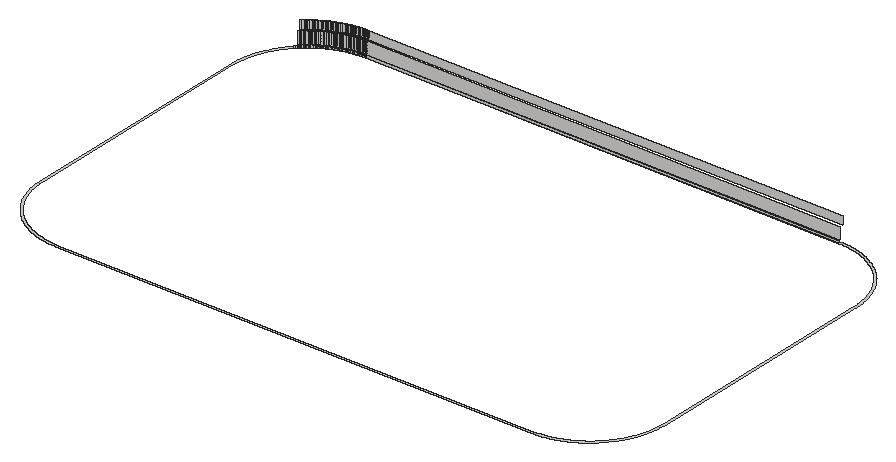
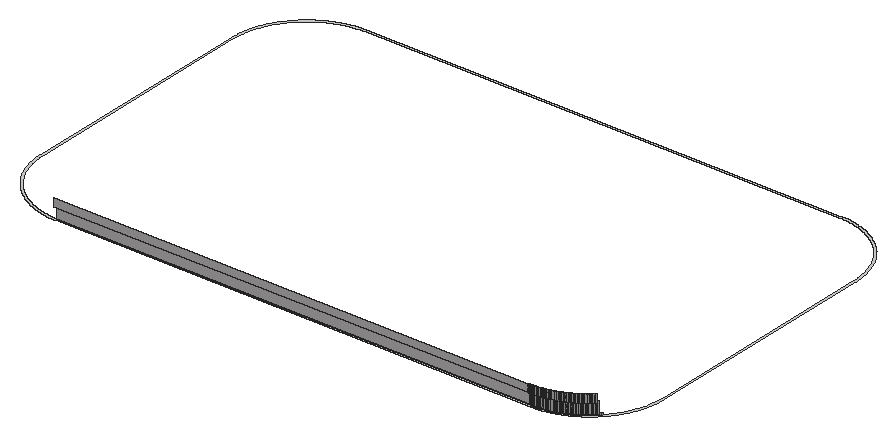
# SketchUp Ruby script. Lengths in inches.
U = 1.inch
M = Sketchup.active_model
def pt(a) = Geom::Point3d.new(a.map { |v| v * U })
def face(e, loops, mat)
  f = e.add_face(loops[0].map { |a| pt(a) })
  loops[1..].each { |l| e.add_face(l.map { |a| pt(a) }).erase! }
  f.material = f.back_material = mat if mat
  f
end
# faces: each face lists its corners as indices into pts; further lists are holes
def faces(e, pts, list, mat = nil) = list.each { |f| face(e, (f[0].is_a?(Array) ? f : [f]).map { |l| l.map { |i| pts[i] } }, mat) }
# xy, xz, yz: faces in a plane at the given z, y or x. An outline is a flat list of corners, or four numbers for a rectangle; further outlines are holes
def ring(l) = l.size == 4 ? [[l[0], l[1]], [l[2], l[1]], [l[2], l[3]], [l[0], l[3]]] : l.each_slice(2).to_a
def flat(e, list, mat, &to3) = list.each { |f| face(e, (f[0].is_a?(Array) ? f : [f]).map { |l| ring(l).map { |u, v| to3.(u, v) } }, mat) }
def xy(e, z, list, mat = nil) = flat(e, list, mat) { |x, y| [x, y, z] }
def xz(e, y, list, mat = nil) = flat(e, list, mat) { |x, z| [x, y, z] }
def yz(e, x, list, mat = nil) = flat(e, list, mat) { |y, z| [x, y, z] }
def lines(e, pts, list) = list.each { |a, b| e.add_line(pt(pts[a]), pt(pts[b])) }
# prism: a flat outline (further loops are holes) pulled along v
def prism(e, loops, v, mat = nil)
  f = face(e, loops, mat); d = Geom::Vector3d.new(v.map { |x| x * U })
  f.pushpull(f.normal.samedirection?(d) ? d.length : -d.length)
end
def box(e, o, s, mat = nil) = prism(e, [[o, [o[0] + s[0], o[1], o[2]], [o[0] + s[0], o[1] + s[1], o[2]], [o[0], o[1] + s[1], o[2]]]], [0, 0, s[2]], mat)
def at(x, y, z, deg = 0) = Geom::Transformation.translation(pt([x, y, z])) * Geom::Transformation.rotation(ORIGIN, Z_AXIS, deg.degrees)
def axes(o, x, y, z) = Geom::Transformation.new([*x, 0, *y, 0, *z, 0, *pt(o).to_a, 1])
def part(name) = M.definitions.add(name)
# library, detail: a bought-in or finely detailed component or shape, given as its bounding box
def library(name, o, s) = part(name).tap { |d| box(d.entities, o, s) }
def detail(e, o, s) = box(e.add_group.entities, o, s)
def put(e, d, t, mat = nil) = e.add_instance(d, t).tap { |i| i.material = mat if mat }
def group(e, t, mat = nil) = e.add_group.tap { |g| g.transformation = t; g.material = mat if mat }.entities
root = M.entities
M.materials.add("[Quartz Light Brown]").color = [215, 212, 212]
xy(root,486,[[[224.5,282.7,464.5,282.7,464.99,282.71,465.99,282.75,466.49,282.78,466.98,282.82,467.48,282.86,467.97,282.91,468.47,282.96,468.96,283.03,469.45,283.09,469.94,283.17,470.44,283.25,470.92,283.34,471.41,283.43,471.9,283.53,472.39,283.64,472.87,283.75,473.35,283.87,473.84,284,474.31,284.13,475.27,284.41,475.74,284.5625,476.21,284.72,476.68,284.88,477.62,285.22,478.08,285.41,478.54,285.59,479.46,285.99,479.91,286.19,480.36,286.4,480.81,286.62,481.25,286.84,481.69,287.07,482.57,287.55,483,287.79,483.43,288.04,483.85,288.3,484.28,288.5625,484.7,288.83,485.11,289.11,485.52,289.38,486.34,289.96,486.74,290.25,487.13,290.55,487.53,290.86,487.91,291.17,488.3,291.49,489.06,292.13,489.43,292.46,489.79,292.8,490.16,293.14,490.52,293.48,491.22,294.18,491.5625,294.54,491.9,294.91,492.24,295.27,492.57,295.65,492.9,296.02,493.22,296.4,494.15,297.57,494.45,297.96,494.74,298.37,495.03,298.77,495.32,299.18,495.6,299.59,495.87,300,496.14,300.42,496.4,300.85,496.66,301.27,496.91,301.7,497.15,302.13,497.4,302.57,497.86,303.45,498.08,303.89,498.3,304.34,498.51,304.79,498.71,305.25,498.91,305.7,499.11,306.16,499.29,306.62,499.48,307.08,499.82,308.02,500.14,308.96,500.29,309.43,500.44,309.91,500.57,310.39,500.71,310.87,500.95,311.83,501.0625,312.31,501.17,312.8,501.27,313.29,501.45,314.27,501.61,315.25,501.67,315.74,501.74,316.23,501.79,316.73,501.84,317.22,501.92,318.22,501.95,318.71,501.99,319.71,502,320.2,502,441.2,501.99,441.7,501.97,442.19,501.95,442.69,501.92,443.1875,501.88,443.68,501.84,444.18,501.79,444.67,501.74,445.17,501.67,445.66,501.61,446.15,501.53,446.65,501.45,447.14,501.27,448.11,501.17,448.6,501.0625,449.09,500.95,449.57,500.83,450.05,500.71,450.54,500.57,451.02,500.44,451.49,500.29,451.97,500.14,452.44,499.98,452.92,499.82,453.39,499.65,453.85,499.48,454.32,499.29,454.78,499.11,455.24,498.71,456.16,498.51,456.61,498.3,457.06,498.08,457.51,497.86,457.95,497.4,458.83,497.15,459.27,496.91,459.7,496.66,460.13,496.4,460.56,496.14,460.98,495.87,461.4,495.6,461.8125,495.32,462.22,494.74,463.04,494.45,463.4375,494.15,463.83,493.84,464.23,493.53,464.62,493.22,465,492.9,465.38,492.57,465.76,492.24,466.13,491.9,466.5,491.5625,466.86,491.22,467.22,490.52,467.92,490.16,468.27,489.79,468.61,489.43,468.94,489.06,469.27,488.68,469.6,488.3,469.92,487.91,470.23,487.53,470.54,487.13,470.85,486.74,471.15,486.34,471.44,485.52,472.02,485.11,472.3,484.7,472.57,484.28,472.84,483.85,473.1,483.43,473.36,482.57,473.86,482.13,474.1,481.25,474.56,480.81,474.78,480.36,475,479.46,475.42,479,475.62,478.08,476,477.62,476.18,476.68,476.52,475.74,476.84,475.27,476.99,474.79,477.14,474.31,477.27,473.84,477.41,473.35,477.53,472.87,477.65,472.39,477.76,471.9,477.87,471.41,477.97,470.92,478.06,470.44,478.15,469.94,478.23,469.45,478.31,468.96,478.375,468.47,478.4375,467.97,478.49,467.48,478.54,466.98,478.58,466.49,478.62,465.99,478.65,465.49,478.67,464.99,478.6875,464.5,478.7,224.5,478.7,224.01,478.6875,223.51,478.67,223.01,478.65,222.51,478.62,222.02,478.58,221.52,478.54,221.03,478.49,220.53,478.4375,220.04,478.375,219.55,478.31,219.06,478.23,218.56,478.15,218.08,478.06,217.59,477.97,217.1,477.87,216.61,477.76,216.13,477.65,215.65,477.53,215.16,477.41,214.69,477.27,214.21,477.14,213.73,476.99,213.26,476.84,212.32,476.52,211.38,476.18,210.92,476,210,475.62,209.54,475.42,208.64,475,208.19,474.78,207.75,474.56,206.87,474.1,206.43,473.86,205.57,473.36,205.15,473.1,204.72,472.84,204.3,472.57,203.89,472.3,203.48,472.02,202.66,471.44,202.26,471.15,201.87,470.85,201.47,470.54,201.09,470.23,200.7,469.92,200.32,469.6,199.94,469.27,199.57,468.94,199.21,468.61,198.84,468.27,198.48,467.92,197.78,467.22,197.4375,466.86,197.1,466.5,196.76,466.13,196.43,465.76,196.1,465.38,195.78,465,195.47,464.62,195.16,464.23,194.85,463.83,194.55,463.4375,194.26,463.04,193.68,462.22,193.4,461.8125,193.13,461.4,192.86,460.98,192.6,460.56,192.34,460.13,192.09,459.7,191.85,459.27,191.6,458.83,191.14,457.95,190.92,457.51,190.7,457.06,190.49,456.61,190.29,456.16,189.89,455.24,189.71,454.78,189.52,454.32,189.35,453.85,189.18,453.39,189.02,452.92,188.86,452.44,188.71,451.97,188.56,451.49,188.43,451.02,188.29,450.54,188.17,450.05,188.05,449.57,187.9375,449.09,187.83,448.6,187.73,448.11,187.55,447.14,187.47,446.65,187.39,446.15,187.33,445.66,187.26,445.17,187.21,444.67,187.16,444.18,187.12,443.68,187.08,443.1875,187.05,442.69,187.03,442.19,187.01,441.7,187,441.2,187,320.2,187.01,319.71,187.05,318.71,187.08,318.22,187.16,317.22,187.21,316.73,187.26,316.23,187.33,315.74,187.39,315.25,187.55,314.27,187.73,313.29,187.83,312.8,187.9375,312.31,188.05,311.83,188.29,310.87,188.43,310.39,188.56,309.91,188.71,309.43,188.86,308.96,189.18,308.02,189.52,307.08,189.71,306.62,189.89,306.16,190.09,305.7,190.29,305.25,190.49,304.79,190.7,304.34,190.92,303.89,191.14,303.45,191.6,302.57,191.85,302.13,192.09,301.7,192.34,301.27,192.6,300.85,192.86,300.42,193.13,300,193.4,299.59,193.68,299.18,193.97,298.77,194.26,298.37,194.55,297.96,194.85,297.57,195.78,296.4,196.1,296.02,196.43,295.65,196.76,295.27,197.1,294.91,197.4375,294.54,197.78,294.18,198.48,293.48,198.84,293.14,199.21,292.8,199.57,292.46,199.94,292.13,200.7,291.49,201.09,291.17,201.47,290.86,201.87,290.55,202.26,290.25,202.66,289.96,203.48,289.38,203.89,289.11,204.3,288.83,204.72,288.5625,205.15,288.3,205.57,288.04,206,287.79,206.43,287.55,207.31,287.07,207.75,286.84,208.19,286.62,208.64,286.4,209.09,286.19,209.54,285.99,210.46,285.59,210.92,285.41,211.38,285.22,212.32,284.88,212.79,284.72,213.26,284.5625,213.73,284.41,214.69,284.13,215.16,284,215.65,283.87,216.13,283.75,216.61,283.64,217.1,283.53,217.59,283.43,218.08,283.34,218.56,283.25,219.06,283.17,219.55,283.09,220.04,283.03,220.53,282.96,221.03,282.91,221.52,282.86,222.02,282.82,222.51,282.78,223.01,282.75,224.01,282.71],[224.52,283.7,224.03,283.71,223.55,283.73,223.0625,283.75,222.58,283.78,222.1,283.82,221.61,283.86,221.13,283.9,219.69,284.08,218.73,284.24,218.26,284.32,217.78,284.41,217.31,284.51,216.83,284.61,216.36,284.72,215.42,284.96,214.96,285.09,214.49,285.22,214.03,285.37,213.57,285.51,213.11,285.66,212.65,285.82,212.19,285.99,211.74,286.16,210.84,286.52,210.39,286.71,209.95,286.9,209.51,287.1,209.07,287.31,208.64,287.52,208.2,287.73,207.77,287.96,207.35,288.18,206.92,288.42,206.08,288.9,205.67,289.15,204.85,289.67,204.44,289.9375,204.04,290.21,203.65,290.49,203.25,290.77,202.86,291.05,202.48,291.35,202.09,291.64,201.72,291.95,201.34,292.25,200.97,292.57,200.6,292.88,200.24,293.2,199.88,293.53,199.53,293.86,199.18,294.2,198.5,294.88,198.16,295.23,197.83,295.59,197.5,295.94,197.18,296.31,196.86,296.67,196.55,297.04,196.25,297.42,195.94,297.79,195.65,298.18,195.35,298.5625,195.07,298.95,194.78,299.35,194.51,299.74,194.24,300.14,193.97,300.55,193.45,301.37,193.2,301.78,192.72,302.62,192.48,303.05,192.26,303.47,192.03,303.9,191.82,304.34,191.6,304.77,191.2,305.65,191,306.1,190.82,306.54,190.63,306.99,190.29,307.89,190.12,308.35,189.96,308.81,189.8125,309.27,189.66,309.73,189.52,310.19,189.39,310.66,189.26,311.125,189.14,311.59,189.02,312.0625,188.91,312.54,188.71,313.48,188.53,314.44,188.46,314.91,188.38,315.39,188.2,316.83,188.16,317.32,188.11,317.8,188.05,318.76,188.03,319.25,188.01,319.73,188,320.22,188,441.19,188.01,441.67,188.03,442.15,188.05,442.64,188.11,443.6,188.16,444.09,188.2,444.57,188.38,446.01,188.46,446.49,188.53,446.97,188.62,447.44,188.71,447.92,188.81,448.39,188.91,448.87,189.02,449.34,189.26,450.28,189.39,450.74,189.52,451.21,189.66,451.67,189.8125,452.13,189.96,452.59,190.12,453.05,190.29,453.51,190.63,454.41,190.82,454.86,191,455.31,191.6,456.63,191.82,457.07,192.03,457.5,192.26,457.93,192.48,458.36,193.2,459.62,193.45,460.03,193.97,460.85,194.24,461.26,194.78,462.06,195.07,462.45,195.35,462.84,195.65,463.23,195.94,463.61,196.25,463.99,196.55,464.36,196.86,464.73,197.18,465.1,197.5,465.46,197.83,465.82,198.16,466.17,198.5,466.52,199.18,467.2,199.53,467.54,199.88,467.87,200.24,468.2,200.6,468.52,200.97,468.84,201.34,469.15,201.72,469.46,202.09,469.76,202.48,470.06,202.86,470.35,203.25,470.63,203.65,470.92,204.04,471.19,204.44,471.47,205.67,472.25,206.08,472.5,206.92,472.98,207.35,473.22,207.77,473.45,208.2,473.67,208.64,473.89,209.07,474.1,210.39,474.7,210.84,474.88,211.29,475.07,212.19,475.41,212.65,475.58,213.11,475.74,214.03,476.04,214.49,476.18,214.96,476.3125,215.42,476.44,215.89,476.5625,216.36,476.68,216.83,476.79,217.31,476.89,217.78,476.99,218.26,477.08,218.73,477.17,219.21,477.25,219.69,477.32,221.13,477.5,221.61,477.55,222.1,477.59,222.58,477.62,223.0625,477.65,223.55,477.67,224.03,477.6875,224.52,477.7,464.48,477.7,464.97,477.6875,465.45,477.67,465.9375,477.65,466.42,477.62,466.9,477.59,467.39,477.55,467.87,477.5,469.31,477.32,469.79,477.25,470.27,477.17,470.74,477.08,471.22,476.99,471.69,476.89,472.17,476.79,472.64,476.68,473.11,476.5625,473.58,476.44,474.04,476.3125,474.51,476.18,474.97,476.04,475.89,475.74,476.35,475.58,476.81,475.41,477.71,475.07,478.16,474.88,478.61,474.7,479.93,474.1,480.36,473.89,480.8,473.67,481.23,473.45,481.65,473.22,482.08,472.98,482.92,472.5,483.33,472.25,484.56,471.47,484.96,471.19,485.35,470.92,485.75,470.63,486.14,470.35,486.52,470.06,486.91,469.76,487.28,469.46,487.66,469.15,488.03,468.84,488.4,468.52,488.76,468.2,489.12,467.87,489.47,467.54,489.82,467.2,490.5,466.52,490.84,466.17,491.17,465.82,491.5,465.46,491.82,465.1,492.14,464.73,492.45,464.36,492.75,463.99,493.06,463.61,493.35,463.23,493.65,462.84,493.93,462.45,494.22,462.06,494.76,461.26,495.03,460.85,495.55,460.03,495.8,459.62,496.52,458.36,496.74,457.93,496.97,457.5,497.18,457.07,497.4,456.63,498,455.31,498.18,454.86,498.37,454.41,498.71,453.51,498.88,453.05,499.04,452.59,499.1875,452.13,499.34,451.67,499.48,451.21,499.61,450.74,499.74,450.28,499.98,449.34,500.09,448.87,500.19,448.39,500.29,447.92,500.38,447.44,500.47,446.97,500.54,446.49,500.62,446.01,500.8,444.57,500.84,444.09,500.89,443.6,500.95,442.64,500.97,442.15,500.99,441.67,501,441.19,501,320.22,500.99,319.73,500.97,319.25,500.95,318.76,500.89,317.8,500.84,317.32,500.8,316.83,500.62,315.39,500.54,314.91,500.47,314.44,500.29,313.48,500.09,312.54,499.98,312.0625,499.86,311.59,499.74,311.125,499.61,310.66,499.48,310.19,499.34,309.73,499.1875,309.27,499.04,308.81,498.88,308.35,498.71,307.89,498.37,306.99,498.18,306.54,498,306.1,497.8,305.65,497.4,304.77,497.18,304.34,496.97,303.9,496.74,303.47,496.52,303.05,496.28,302.62,495.8,301.78,495.55,301.37,495.03,300.55,494.76,300.14,494.49,299.74,494.22,299.35,493.93,298.95,493.65,298.5625,493.35,298.18,493.06,297.79,492.75,297.42,492.45,297.04,492.14,296.67,491.82,296.31,491.5,295.94,491.17,295.59,490.84,295.23,490.5,294.88,489.82,294.2,489.47,293.86,489.12,293.53,488.76,293.2,488.4,292.88,488.03,292.57,487.66,292.25,487.28,291.95,486.91,291.64,486.52,291.35,486.14,291.05,485.75,290.77,485.35,290.49,484.96,290.21,484.56,289.9375,484.15,289.67,483.33,289.15,482.92,288.9,482.08,288.42,481.65,288.18,481.23,287.96,480.8,287.73,480.36,287.52,479.93,287.31,479.49,287.1,479.05,286.9,478.61,286.71,478.16,286.52,477.26,286.16,476.81,285.99,476.35,285.82,475.89,285.66,475.43,285.51,474.97,285.37,474.51,285.22,474.04,285.09,473.58,284.96,472.64,284.72,472.17,284.61,471.69,284.51,471.22,284.41,470.74,284.32,470.27,284.24,469.31,284.08,467.87,283.9,467.39,283.86,466.9,283.82,466.42,283.78,465.9375,283.75,465.45,283.73,464.97,283.71,464.48,283.7]]],"[Quartz Light Brown]")
xz(root,477.7,[[224.52,486,225,487],[225,486,464,487]],"[Quartz Light Brown]")
xz(root,478.7,[[224.5,487,225,493],[225,487,464,493]],"[Quartz Light Brown]")
xz(root,480.2,[[224.48,493,225,497],[225,493,464,497]],"[Quartz Light Brown]")
p = [[198.5,466.52,486],[198.16,466.17,486],[198.16,466.17,487],[198.5,466.52,487],[198.84,466.86,486],[198.84,466.86,487],
  [199.18,467.2,486],[199.18,467.2,487],[199.53,467.54,486],[199.53,467.54,487],[199.88,467.87,486],[199.88,467.87,487],
  [200.24,468.2,486],[200.24,468.2,487],[200.6,468.52,486],[200.6,468.52,487],[200.97,468.84,486],[200.97,468.84,487],
  [201.34,469.15,486],[201.34,469.15,487],[201.72,469.46,486],[201.72,469.46,487],[202.09,469.76,486],[202.09,469.76,487],
  [202.48,470.06,486],[202.48,470.06,487],[202.86,470.35,486],[202.86,470.35,487],[203.25,470.63,486],[203.25,470.63,487],
  [203.65,470.92,486],[203.65,470.92,487],[204.04,471.19,486],[204.04,471.19,487],[204.44,471.47,486],[204.44,471.47,487],
  [204.85,471.73,486],[204.85,471.73,487],[205.26,471.99,486],[205.26,471.99,487],[205.67,472.25,486],[205.67,472.25,487],
  [206.08,472.5,486],[206.08,472.5,487],[206.5,472.74,486],[206.5,472.74,487],[206.92,472.98,486],[206.92,472.98,487],
  [207.35,473.22,486],[207.35,473.22,487],[207.77,473.45,486],[207.77,473.45,487],[208.2,473.67,486],[208.2,473.67,487],
  [208.64,473.89,486],[208.64,473.89,487],[209.07,474.1,486],[209.07,474.1,487],[209.51,474.3,486],[209.51,474.3,487],
  [209.95,474.5,486],[209.95,474.5,487],[210.39,474.7,486],[210.39,474.7,487],[210.84,474.88,486],[210.84,474.88,487],
  [211.29,475.07,486],[211.29,475.07,487],[211.74,475.24,486],[211.74,475.24,487],[212.19,475.41,486],[212.19,475.41,487],
  [212.65,475.58,486],[212.65,475.58,487],[213.11,475.74,486],[213.11,475.74,487],[213.57,475.89,486],[213.57,475.89,487],
  [214.03,476.04,486],[214.03,476.04,487],[214.49,476.18,486],[214.49,476.18,487],[214.96,476.3125,486],[214.96,476.3125,487],
  [215.42,476.44,486],[215.42,476.44,487],[215.89,476.5625,486],[215.89,476.5625,487],[216.36,476.68,486],[216.36,476.68,487],
  [216.83,476.79,486],[216.83,476.79,487],[217.31,476.89,486],[217.31,476.89,487],[217.78,476.99,486],[217.78,476.99,487],
  [218.26,477.08,486],[218.26,477.08,487],[218.73,477.17,486],[218.73,477.17,487],[219.21,477.25,486],[219.21,477.25,487],
  [219.69,477.32,486],[219.69,477.32,487],[220.17,477.38,486],[220.17,477.38,487],[220.65,477.44,486],[220.65,477.44,487],
  [221.13,477.5,486],[221.13,477.5,487],[221.61,477.55,486],[221.61,477.55,487],[222.1,477.59,486],[222.1,477.59,487],
  [222.58,477.62,486],[222.58,477.62,487],[223.0625,477.65,486],[223.0625,477.65,487],[223.55,477.67,486],[223.55,477.67,487],
  [224.03,477.6875,486],[224.03,477.6875,487],[224.52,477.7,486],[224.52,477.7,487],[198.48,467.92,487],[198.48,467.92,493],
  [198.84,468.27,493],[198.84,468.27,487],[199.21,468.61,493],[199.21,468.61,487],[199.57,468.94,493],[199.57,468.94,487],
  [199.94,469.27,493],[199.94,469.27,487],[200.32,469.6,493],[200.32,469.6,487],[200.7,469.92,493],[200.7,469.92,487],
  [201.09,470.23,493],[201.09,470.23,487],[201.47,470.54,493],[201.47,470.54,487],[201.87,470.85,493],[201.87,470.85,487],
  [202.26,471.15,493],[202.26,471.15,487],[202.66,471.44,493],[202.66,471.44,487],[203.07,471.73,493],[203.07,471.73,487],
  [203.48,472.02,493],[203.48,472.02,487],[203.89,472.3,493],[203.89,472.3,487],[204.3,472.57,493],[204.3,472.57,487],
  [204.72,472.84,493],[204.72,472.84,487],[205.15,473.1,493],[205.15,473.1,487],[205.57,473.36,493],[205.57,473.36,487],
  [206,473.61,493],[206,473.61,487],[206.43,473.86,493],[206.43,473.86,487],[206.87,474.1,493],[206.87,474.1,487],
  [207.31,474.33,493],[207.31,474.33,487],[207.75,474.56,493],[207.75,474.56,487],[208.19,474.78,493],[208.19,474.78,487],
  [208.64,475,493],[208.64,475,487],[209.09,475.21,493],[209.09,475.21,487],[209.54,475.42,493],[209.54,475.42,487],
  [210,475.62,493],[210,475.62,487],[210.46,475.81,493],[210.46,475.81,487],[210.92,476,493],[210.92,476,487],
  [211.38,476.18,493],[211.38,476.18,487],[211.85,476.35,493],[211.85,476.35,487],[212.32,476.52,493],[212.32,476.52,487],
  [212.79,476.68,493],[212.79,476.68,487],[213.26,476.84,493],[213.26,476.84,487],[213.73,476.99,493],[213.73,476.99,487],
  [214.21,477.14,493],[214.21,477.14,487],[214.69,477.27,493],[214.69,477.27,487],[215.16,477.41,493],[215.16,477.41,487],
  [215.65,477.53,493],[215.65,477.53,487],[216.13,477.65,493],[216.13,477.65,487],[216.61,477.76,493],[216.61,477.76,487],
  [217.1,477.87,493],[217.1,477.87,487],[217.59,477.97,493],[217.59,477.97,487],[218.08,478.06,493],[218.08,478.06,487],
  [218.56,478.15,493],[218.56,478.15,487],[219.06,478.23,493],[219.06,478.23,487],[219.55,478.31,493],[219.55,478.31,487],
  [220.04,478.375,493],[220.04,478.375,487],[220.53,478.4375,493],[220.53,478.4375,487],[221.03,478.49,493],[221.03,478.49,487],
  [221.52,478.54,493],[221.52,478.54,487],[222.02,478.58,493],[222.02,478.58,487],[222.51,478.62,493],[222.51,478.62,487],
  [223.01,478.65,493],[223.01,478.65,487],[223.51,478.67,493],[223.51,478.67,487],[224.01,478.6875,493],[224.01,478.6875,487],
  [224.5,478.7,493],[224.5,478.7,487],[198.57,470.06,493],[198.1875,469.71,493],[198.1875,469.71,497],[198.57,470.06,497],
  [198.96,470.4,493],[198.96,470.4,497],[199.35,470.74,493],[199.35,470.74,497],[199.74,471.07,493],[199.74,471.07,497],
  [200.14,471.4,493],[200.14,471.4,497],[200.55,471.72,493],[200.55,471.72,497],[200.95,472.04,493],[200.95,472.04,497],
  [201.37,472.35,493],[201.37,472.35,497],[201.78,472.66,493],[201.78,472.66,497],[202.2,472.96,493],[202.2,472.96,497],
  [202.625,473.25,493],[202.625,473.25,497],[203.05,473.54,493],[203.05,473.54,497],[203.49,473.83,493],[203.49,473.83,497],
  [203.92,474.11,493],[203.92,474.11,497],[204.36,474.38,493],[204.36,474.38,497],[204.8,474.65,493],[204.8,474.65,497],
  [205.25,474.91,493],[205.25,474.91,497],[205.7,475.16,493],[205.7,475.16,497],[206.15,475.41,493],[206.15,475.41,497],
  [206.61,475.66,493],[206.61,475.66,497],[207.07,475.9,493],[207.07,475.9,497],[207.53,476.13,493],[207.53,476.13,497],
  [207.99,476.35,493],[207.99,476.35,497],[208.46,476.57,493],[208.46,476.57,497],[208.93,476.79,493],[208.93,476.79,497],
  [209.41,476.99,493],[209.41,476.99,497],[209.88,477.19,493],[209.88,477.19,497],[210.36,477.39,493],[210.36,477.39,497],
  [210.84,477.58,493],[210.84,477.58,497],[211.33,477.76,493],[211.33,477.76,497],[211.81,477.94,493],[211.81,477.94,497],
  [212.3,478.1,493],[212.3,478.1,497],[212.79,478.27,493],[212.79,478.27,497],[213.29,478.42,493],[213.29,478.42,497],
  [213.78,478.57,493],[213.78,478.57,497],[214.28,478.72,493],[214.28,478.72,497],[214.78,478.86,493],[214.78,478.86,497],
  [215.28,478.99,493],[215.28,478.99,497],[215.78,479.11,493],[215.78,479.11,497],[216.28,479.23,493],[216.28,479.23,497],
  [216.79,479.34,493],[216.79,479.34,497],[217.29,479.44,493],[217.29,479.44,497],[217.8,479.54,493],[217.8,479.54,497],
  [218.3125,479.63,493],[218.3125,479.63,497],[218.82,479.71,493],[218.82,479.71,497],[219.33,479.79,493],[219.33,479.79,497],
  [219.84,479.86,493],[219.84,479.86,497],[220.36,479.93,493],[220.36,479.93,497],[220.87,479.98,493],[220.87,479.98,497],
  [221.39,480.04,493],[221.39,480.04,497],[221.9,480.08,493],[221.9,480.08,497],[222.42,480.12,493],[222.42,480.12,497],
  [222.93,480.15,493],[222.93,480.15,497],[223.45,480.17,493],[223.45,480.17,497],[223.97,480.1875,493],[223.97,480.1875,497],
  [224.48,480.2,493],[224.48,480.2,497],[225,478.7,493],[225,478.7,495]]
faces(root,p,[[0,1,2,3],[4,0,3,5],[6,4,5,7],[8,6,7,9],[10,8,9,11],[12,10,11,13],[14,12,13,15],[16,14,15,17],
  [18,16,17,19],[20,18,19,21],[22,20,21,23],[24,22,23,25],[26,24,25,27],[28,26,27,29],[30,28,29,31],[32,30,31,33],
  [34,32,33,35],[36,34,35,37],[38,36,37,39],[40,38,39,41],[42,40,41,43],[44,42,43,45],[46,44,45,47],[48,46,47,49],
  [50,48,49,51],[52,50,51,53],[54,52,53,55],[56,54,55,57],[58,56,57,59],[60,58,59,61],[62,60,61,63],[64,62,63,65],
  [66,64,65,67],[68,66,67,69],[70,68,69,71],[72,70,71,73],[74,72,73,75],[76,74,75,77],[78,76,77,79],[80,78,79,81],
  [82,80,81,83],[84,82,83,85],[86,84,85,87],[88,86,87,89],[90,88,89,91],[92,90,91,93],[94,92,93,95],[96,94,95,97],
  [98,96,97,99],[100,98,99,101],[102,100,101,103],[104,102,103,105],[106,104,105,107],[108,106,107,109],[110,108,109,111],[112,110,111,113],
  [114,112,113,115],[116,114,115,117],[118,116,117,119],[120,118,119,121],[122,120,121,123],[124,125,126,127],[127,126,128,129],[129,128,130,131],
  [131,130,132,133],[133,132,134,135],[135,134,136,137],[137,136,138,139],[139,138,140,141],[141,140,142,143],[143,142,144,145],[145,144,146,147],
  [147,146,148,149],[149,148,150,151],[151,150,152,153],[153,152,154,155],[155,154,156,157],[157,156,158,159],[159,158,160,161],[161,160,162,163],
  [163,162,164,165],[165,164,166,167],[167,166,168,169],[169,168,170,171],[171,170,172,173],[173,172,174,175],[175,174,176,177],[177,176,178,179],
  [179,178,180,181],[181,180,182,183],[183,182,184,185],[185,184,186,187],[187,186,188,189],[189,188,190,191],[191,190,192,193],[193,192,194,195],
  [195,194,196,197],[197,196,198,199],[199,198,200,201],[201,200,202,203],[203,202,204,205],[205,204,206,207],[207,206,208,209],[209,208,210,211],
  [211,210,212,213],[213,212,214,215],[215,214,216,217],[217,216,218,219],[219,218,220,221],[221,220,222,223],[223,222,224,225],[225,224,226,227],
  [227,226,228,229],[229,228,230,231],[231,230,232,233],[233,232,234,235],[235,234,236,237],[237,236,238,239],[239,238,240,241],[242,243,244,245],
  [246,242,245,247],[248,246,247,249],[250,248,249,251],[252,250,251,253],[254,252,253,255],[256,254,255,257],[258,256,257,259],[260,258,259,261],
  [262,260,261,263],[264,262,263,265],[266,264,265,267],[268,266,267,269],[270,268,269,271],[272,270,271,273],[274,272,273,275],[276,274,275,277],
  [278,276,277,279],[280,278,279,281],[282,280,281,283],[284,282,283,285],[286,284,285,287],[288,286,287,289],[290,288,289,291],[292,290,291,293],
  [294,292,293,295],[296,294,295,297],[298,296,297,299],[300,298,299,301],[302,300,301,303],[304,302,303,305],[306,304,305,307],[308,306,307,309],
  [310,308,309,311],[312,310,311,313],[314,312,313,315],[316,314,315,317],[318,316,317,319],[320,318,319,321],[322,320,321,323],[324,322,323,325],
  [326,324,325,327],[328,326,327,329],[330,328,329,331],[332,330,331,333],[334,332,333,335],[336,334,335,337],[338,336,337,339],[340,338,339,341],
  [342,340,341,343],[344,342,343,345],[346,344,345,347],[348,346,347,349],[350,348,349,351],[352,350,351,353],[354,352,353,355]],"[Quartz Light Brown]")
lines(root,p,[[356,357]])
